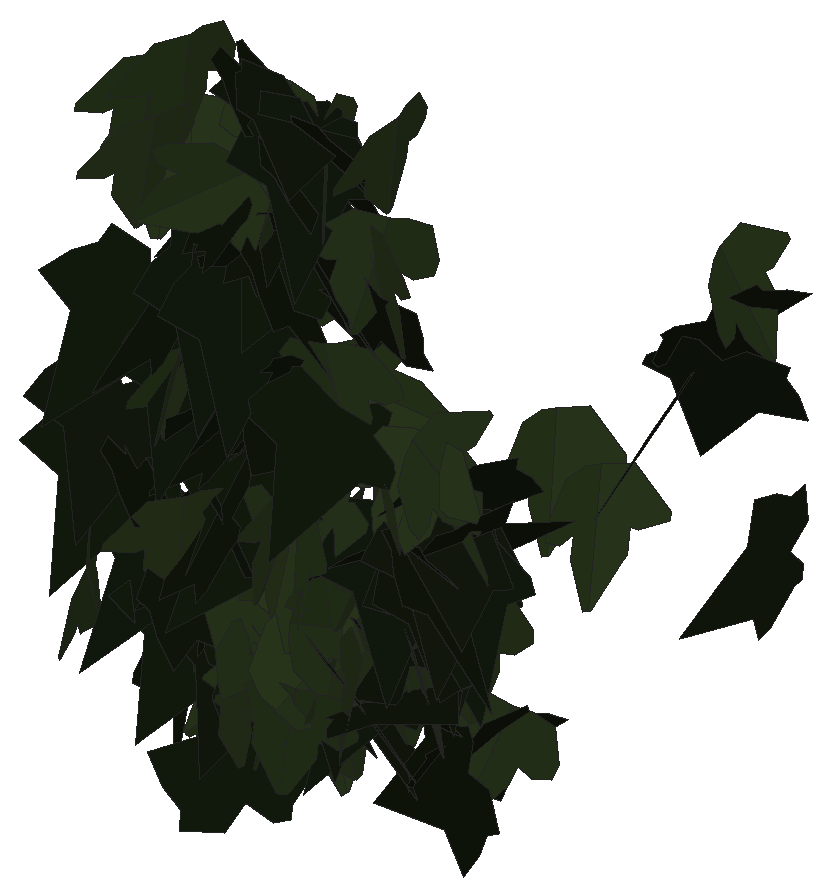
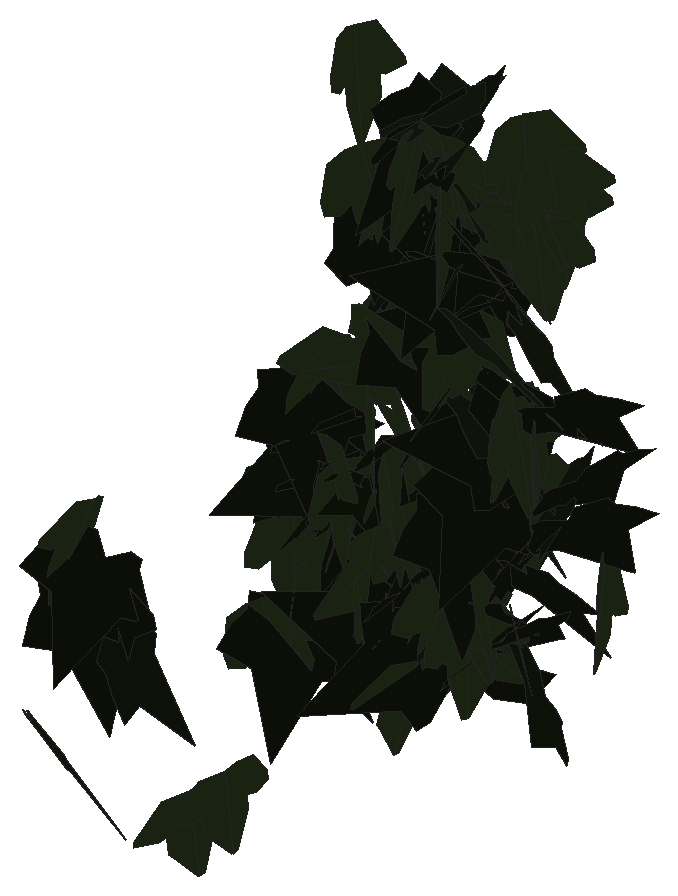
# SketchUp Ruby script. Lengths in inches.
U = 1.inch
M = Sketchup.active_model
def pt(a) = Geom::Point3d.new(a.map { |v| v * U })
def face(e, loops, mat)
  f = e.add_face(loops[0].map { |a| pt(a) })
  loops[1..].each { |l| e.add_face(l.map { |a| pt(a) }).erase! }
  f.material = f.back_material = mat if mat
  f
end
# faces: each face lists its corners as indices into pts; further lists are holes
def faces(e, pts, list, mat = nil) = list.each { |f| face(e, (f[0].is_a?(Array) ? f : [f]).map { |l| l.map { |i| pts[i] } }, mat) }
# xy, xz, yz: faces in a plane at the given z, y or x. An outline is a flat list of corners, or four numbers for a rectangle; further outlines are holes
def ring(l) = l.size == 4 ? [[l[0], l[1]], [l[2], l[1]], [l[2], l[3]], [l[0], l[3]]] : l.each_slice(2).to_a
def flat(e, list, mat, &to3) = list.each { |f| face(e, (f[0].is_a?(Array) ? f : [f]).map { |l| ring(l).map { |u, v| to3.(u, v) } }, mat) }
def xy(e, z, list, mat = nil) = flat(e, list, mat) { |x, y| [x, y, z] }
def xz(e, y, list, mat = nil) = flat(e, list, mat) { |x, z| [x, y, z] }
def yz(e, x, list, mat = nil) = flat(e, list, mat) { |y, z| [x, y, z] }
def lines(e, pts, list) = list.each { |a, b| e.add_line(pt(pts[a]), pt(pts[b])) }
# prism: a flat outline (further loops are holes) pulled along v
def prism(e, loops, v, mat = nil)
  f = face(e, loops, mat); d = Geom::Vector3d.new(v.map { |x| x * U })
  f.pushpull(f.normal.samedirection?(d) ? d.length : -d.length)
end
def box(e, o, s, mat = nil) = prism(e, [[o, [o[0] + s[0], o[1], o[2]], [o[0] + s[0], o[1] + s[1], o[2]], [o[0], o[1] + s[1], o[2]]]], [0, 0, s[2]], mat)
def at(x, y, z, deg = 0) = Geom::Transformation.translation(pt([x, y, z])) * Geom::Transformation.rotation(ORIGIN, Z_AXIS, deg.degrees)
def axes(o, x, y, z) = Geom::Transformation.new([*x, 0, *y, 0, *z, 0, *pt(o).to_a, 1])
def part(name) = M.definitions.add(name)
# library, detail: a bought-in or finely detailed component or shape, given as its bounding box
def library(name, o, s) = part(name).tap { |d| box(d.entities, o, s) }
def detail(e, o, s) = box(e.add_group.entities, o, s)
def put(e, d, t, mat = nil) = e.add_instance(d, t).tap { |i| i.material = mat if mat }
def group(e, t, mat = nil) = e.add_group.tap { |g| g.transformation = t; g.material = mat if mat }.entities
root = M.entities
M.materials.add("efeu1").color = [18, 25, 13]
M.materials.add("efeu2").color = [43, 57, 29]
c1 = part("ivyleaf_9")
p = [[1.54,2.16,1.25],[1.36,2.04,1.19],[-0.21,0.99,0.68],[-0.71,1.11,0.82],[-0.85,0.86,0.67],[-0.8,0.17,0.21],
  [-0.9,-0.01,0.1],[-0.67,-0.16,-0.02],[-0.08,-0.08,-0.05],[-0.03,-0.6,-0.4],[0.65,-0.88,-0.66],[0.83,-0.6,-0.49],
  [1.29,-0.42,-0.43],[1.8125,-0.07,-0.26],[1.21,0.44,0.15]]
faces(c1.entities,p,[[0,1,2,3,4,5,6,7,8,9,10,11,12,13,14]],"efeu1")
c2 = part("ivyleaf_10")
p = [[0,0.5,-0.03],[-0.0625,2.02,-0.43],[-0.19,2.01,-0.46],[-0.54,1.05,-0.29],[-0.52,0.625,-0.18],[-0.83,0.76,-0.28],
  [-1.16,0.64,-0.33],[-1.15,0.33,-0.24],[-0.77,-0.39,0.02],[-0.3,-0.51,0.16],[0.04,-0.48,0.23],[-0.02,2.01,-0.4375],
  [-0.06,2.01,-0.43],[0.04,-0.49,0.23],[0.67,-0.49,0.14],[1.38,0.36,-0.2],[1.375,0.51,-0.24],[0.81,0.65,-0.19],
  [0.62,0.59,-0.15],[0.6,1.09,-0.28],[0.5,1.23,-0.31]]
faces(c2.entities,p,[[0,1,2,3,4,5,6,7,8,9,10],[11,12,0,13,14,15,16,17,18,19,20]],"efeu2")
put(root,c1,axes([45.125,222.38,245.66],[-0.38766,-0.3113,0.05304],[-0.02008,-0.05951,-0.49604],[0.31515,-0.38672,0.03364]))
put(root,c1,axes([45.24,222.48,242.16],[0.00287,0.24206,0.43749],[-0.08751,0.43099,-0.23788],[-0.49227,-0.0752,0.04484]))
put(root,c1,axes([45.08,222.2,244.22],[-0.31267,-0.3897,0.01922],[-0.01187,-0.01511,-0.49963],[0.38999,-0.3129,0.0002]))
put(root,c2,axes([45.15,221.53,243.23],[0.12994,-0.37779,-0.30066],[-0.03557,0.30302,-0.39613],[0.48151,0.12433,0.05187]))
put(root,c1,axes([45.03,222.16,244.73],[-0.14946,-0.4697,0.08394],[0.01749,-0.0933,-0.49091],[0.47682,-0.14381,0.04432]))
put(root,c1,axes([45.55,222.3125,243.43],[-0.48425,-0.08758,-0.08849],[0.09295,-0.01792,-0.49096],[0.08282,-0.49194,0.03364]))
put(root,c2,axes([45.54,221.95,248.12],[-0.1573,-0.47311,0.03769],[0.00614,-0.04173,-0.49822],[0.47457,-0.15628,0.01894]))
put(root,c1,axes([45.38,221.88,244.28],[0.37177,-0.32094,-0.09373],[-0.06614,0.0668,-0.49108],[0.32774,0.37754,0.00721]))
put(root,c2,axes([45.7,222.07,245.29],[0.21508,-0.38398,-0.23728],[-0.05459,0.23878,-0.43589],[0.44806,0.21341,0.06079]))
put(root,c2,axes([45.62,222.12,247.48],[0.44327,0.22883,-0.03391],[-0.0732,0.06922,-0.48975],[-0.21944,0.43914,0.09487]))
put(root,c2,axes([45.74,222.29,245.22],[-0.05903,-0.49638,0.01103],[0.00533,-0.01174,-0.49983],[0.49648,-0.05889,0.00667]))
put(root,c2,axes([45.75,221.68,247.7],[-0.13253,-0.4821,0.00445],[-0.00203,-0.00406,-0.49998],[0.48211,-0.13254,-0.00088]))
put(root,c1,axes([45.5625,222.47,242.6],[-0.22696,0.01463,-0.44528],[0.4344,-0.10371,-0.22482],[-0.09894,-0.48891,0.03437]))
put(root,c1,axes([45.94,221.9,246.1],[-0.41221,0.27163,-0.07936],[0.06022,-0.05282,-0.49354],[-0.27651,-0.41645,0.01083]))
put(root,c1,axes([45.76,222.47,242.68],[-0.23718,-0.41431,0.14863],[0.02717,-0.18229,-0.46479],[0.43933,-0.2124,0.10898]))
put(root,c2,axes([45.93,221.93,248.46],[-0.16446,-0.47135,-0.02792],[0.01134,0.02562,-0.49921],[0.47204,-0.16483,0.00227]))
put(root,c2,axes([45.79,222.16,247.61],[0.45358,0.20748,0.03487],[0.03418,0.0091,-0.49875],[-0.20759,0.45483,-0.00592]))
put(root,c1,axes([45.875,222.17,245.54],[-0.39092,-0.19237,-0.24531],[0.24802,0.04645,-0.43166],[0.18886,-0.45917,0.05911]))
put(root,c2,axes([45.9,222.18,245.3125],[0.07023,-0.46333,-0.17432],[0.09002,0.18509,-0.45567],[0.48679,0.03262,0.10942]))
put(root,c2,axes([46.25,222.57,243.09],[-0.28832,0.05676,0.40453],[-0.39048,0.10714,-0.29334],[-0.11998,-0.48508,-0.01746]))
put(root,c1,axes([46.34,222.36,246.19],[-0.38197,0.30566,0.1033],[-0.12891,0.00218,-0.48309],[-0.29577,-0.39569,0.07714]))
put(root,c1,axes([45.9,221.86,243.44],[0.25463,-0.22596,-0.3662],[-0.18364,0.32775,-0.32993],[0.38915,0.30252,0.08392]))
put(root,c2,axes([46.11,221.66,244.11],[-0.24677,-0.43476,-0.00936],[0.00286,0.00914,-0.49991],[0.43485,-0.24678,-0.00203]))
put(root,c2,axes([46.12,222.66,242.8125],[-0.20305,-0.45486,-0.0433],[0.02949,0.03424,-0.49795],[0.45596,-0.20477,0.01293]))
put(root,c1,axes([46.14,222.26,244.25],[0.17083,0.45348,0.12318],[0.04347,0.11525,-0.48459],[-0.4679,0.17627,-0.00005]))
put(root,c1,axes([46.05,222.61,242.41],[-0.08781,-0.44591,0.20846],[0.00845,-0.21308,-0.45224],[0.49216,-0.0759,0.04495]))
put(root,c2,axes([46.16,226.73,242.65],[0.15622,0.46568,-0.09349],[-0.04238,-0.08436,-0.49101],[-0.47308,0.16133,0.01311]))
put(root,c1,axes([46.51,222.05,245.05],[-0.37045,0.32819,-0.07112],[0.0024,-0.1033,-0.48921],[-0.3358,-0.3628,0.07496]))
put(root,c2,axes([46.57,221.68,247.53],[0.27567,0.13123,-0.39596],[-0.41325,0.02121,-0.28067],[-0.05687,0.482,0.12016]))
put(root,c1,axes([46.03,222.02,244.69],[0.24987,0.03001,0.43205],[0.35568,0.27036,-0.22449],[-0.24709,0.41953,0.11376]))
put(root,c2,axes([46.5,222.46,242.52],[-0.1614,-0.27023,0.38849],[-0.1581,-0.35609,-0.31337],[0.44604,-0.224,0.0295]))
put(root,c1,axes([46.58,221.7,244.21],[-0.41189,0.28046,-0.04105],[0.03643,-0.01943,-0.49829],[-0.2811,-0.41348,-0.00443]))
put(root,c1,axes([46.625,221.86,247.375],[-0.37652,0.32747,0.03162],[-0.02185,0.02306,-0.49899],[-0.32826,-0.37714,-0.00305]))
put(root,c1,axes([46.47,222.29,243.75],[0.08376,0.48732,-0.0742],[-0.01901,-0.07201,-0.49442],[-0.49257,0.08565,0.00647]))
put(root,c2,axes([46.4,222.65,242.98],[-0.34952,-0.35193,-0.06307],[0.0779,0.01113,-0.49377],[0.34895,-0.35499,0.04705]))
put(root,c2,axes([46.36,222.15,242.64],[-0.3735,0.31157,-0.11585],[0.07852,-0.08663,-0.48614],[-0.323,-0.38134,0.01579]))
put(root,c1,axes([46.375,222.57,242.81],[-0.32423,-0.35122,-0.14671],[0.12402,0.08472,-0.47691],[0.35985,-0.34564,0.03218]))
put(root,c1,axes([46.3125,222.01,246.38],[-0.10842,-0.48688,0.03449],[0.01245,-0.03808,-0.49839],[0.48795,-0.10721,0.02038]))
put(root,c1,axes([46.79,222.1,247.15],[-0.47088,0.16808,0.00458],[-0.00322,0.00463,-0.49997],[-0.16811,-0.47088,-0.00328]))
put(root,c2,axes([46.49,222.27,246.1],[-0.44192,-0.17527,-0.15488],[0.15416,0.03071,-0.47465],[0.17589,-0.46727,0.0269]))
put(root,c1,axes([46.32,222.22,243.91],[0.37188,-0.33039,-0.05049],[-0.03501,0.03661,-0.49743],[0.33238,0.3735,0.0041]))
put(root,c1,axes([46.71,221.77,241.53],[-0.46663,-0.08066,0.16047],[0.15811,0.0274,0.47355],[-0.08518,0.49269,-0.00007]))
put(root,c1,axes([46.81,222.09,244.27],[-0.46675,-0.1788,0.01334],[-0.01132,-0.00773,-0.49981],[0.17894,-0.46687,0.00316]))
put(root,c2,axes([46.62,226.76,242.25],[0.17252,0.46016,-0.09213],[-0.05885,-0.07617,-0.49065],[-0.46559,0.18014,0.02788]))
put(root,c1,axes([46.78,222.23,246.78],[-0.44314,-0.22095,-0.06932],[0.0776,-0.00068,-0.49394],[0.21818,-0.44853,0.03489]))
put(root,c2,axes([46.74,222.49,242.58],[-0.00841,0.42234,-0.2675],[-0.11132,-0.2624,-0.4108],[-0.48738,0.05265,0.09845]))
put(root,c1,axes([46.61,221.9375,246.36],[-0.08779,-0.49219,0.00671],[0.00137,-0.00706,-0.49995],[0.49223,-0.08777,0.00259]))
put(root,c1,axes([46.43,222.0625,246.41],[0.23802,-0.01532,0.43944],[0.38697,0.2446,-0.20107],[-0.20881,0.43582,0.12829]))
put(root,c1,axes([46.54,222.49,242.83],[0.38172,-0.27841,-0.16365],[-0.09931,0.1399,-0.46964],[0.30729,0.39105,0.0515]))
put(root,c2,axes([46.68,222.94,242.11],[0.12285,0.4826,0.04481],[0.00308,0.04545,-0.49792],[-0.48466,0.12262,0.00819]))
put(root,c2,axes([46.77,222.27,247.44],[0.1814,-0.44126,-0.14962],[0.03193,0.17196,-0.46841],[0.46484,0.16039,0.09057]))
put(root,c1,axes([46.72,221.94,246.99],[0.40306,0.29273,-0.04303],[-0.04329,-0.01359,-0.49794],[-0.29269,0.40512,0.01439]))
put(root,c2,axes([46.81,221.47,242.71],[0.11259,-0.12417,-0.47107],[0.05349,0.48371,-0.11472],[0.48421,-0.02456,0.1222]))
put(root,c2,axes([46.95,221.8,244.16],[0.35532,-0.25677,-0.24046],[-0.18313,0.1568,-0.43804],[0.30036,0.39935,0.01738]))
put(root,c1,axes([46.55,222.88,242.36],[0.37762,0.19109,0.26625],[0.24386,0.10753,-0.42305],[-0.21894,0.44936,-0.01199]))
put(root,c1,axes([46.59,221.92,248.5],[0.36501,-0.33331,-0.0753],[-0.04206,0.06552,-0.4939],[0.33911,0.36689,0.01979]))
put(root,c2,axes([46.8,222.15,248.11],[0.49516,-0.06937,-0.00223],[-0.00279,-0.00384,-0.49998],[0.06935,0.49515,-0.00419]))
put(root,c2,axes([46.59,221.97,243.38],[-0.24818,-0.17193,-0.39856],[0.42152,0.01409,-0.26855],[0.10358,-0.4693,0.13795]))
put(root,c1,axes([46.73,222.1875,245.24],[0.2571,-0.3921,-0.17365],[-0.09116,0.14787,-0.46886],[0.41903,0.27275,0.00454]))
put(root,c2,axes([46.99,222.6,243.63],[-0.17064,-0.46105,0.09119],[0.00281,-0.09801,-0.49029],[0.46997,-0.16681,0.03604]))
put(root,c1,axes([46.8,222,246.73],[0.36307,-0.31106,-0.14636],[-0.11129,0.09506,-0.4781],[0.32526,0.37974,-0.0002]))
put(root,c1,axes([47.19,222.11,245.75],[0.07986,0.44036,-0.22294],[-0.08151,-0.21097,-0.44592],[-0.4868,0.10757,0.03809]))
put(root,c2,axes([47.22,221.82,242.55],[-0.43911,-0.21466,0.10538],[-0.09298,-0.04972,-0.48876],[0.22031,-0.44883,0.00375]))
put(root,c2,axes([47.125,222.5,242.27],[-0.16151,-0.44852,-0.15081],[0.05772,0.13948,-0.47667],[0.46966,-0.17138,0.00672]))
put(root,c1,axes([46.96,222.73,242.94],[-0.00201,-0.49969,0.01762],[0.00168,-0.01763,-0.49969],[0.49999,-0.00195,0.00175]))
put(root,c2,axes([47.19,221.84,244.55],[0.07256,-0.47846,0.12574],[0.00556,-0.12629,-0.48376],[0.49468,0.0716,-0.013]))
put(root,c2,axes([47.22,222.2,247.92],[0.02177,-0.42929,-0.25541],[0.04832,0.25627,-0.42661],[0.49718,-0.00611,0.05265]))
put(root,c2,axes([47.25,222.55,244.16],[0.14391,-0.47643,-0.04806],[0.00429,0.05146,-0.49733],[0.47882,0.14272,0.0189]))
put(root,c2,axes([47.29,222.41,242.8],[0.15196,-0.4738,-0.04919],[0.01479,0.0563,-0.4966],[0.47612,0.14947,0.03112]))
put(root,c2,axes([47.32,222.89,242.86],[0.13243,-0.47499,-0.08272],[0.00013,0.08582,-0.49258],[0.48214,0.13044,0.02285]))
put(root,c1,axes([47.04,222.91,242.53],[0.23949,-0.43726,-0.03809],[0.01293,0.0504,-0.49729],[0.43872,0.2372,0.03545]))
put(root,c1,axes([47.09,222.04,248.3125],[-0.12571,-0.43276,0.21661],[0.23524,-0.25022,-0.36339],[0.42292,0.01055,0.26651]))
put(root,c2,axes([47.15,221.86,244.21],[0.44446,-0.15156,0.17172],[0.1627,-0.05492,-0.46959],[0.1612,0.4733,0.00049]))
put(root,c2,axes([47.22,222.72,243.29],[-0.04241,-0.21685,-0.44853],[0.20092,0.40448,-0.21455],[0.45589,-0.19843,0.05283]))
put(root,c1,axes([47.17,221.7,248.07],[0.40828,-0.18027,-0.22542],[-0.15091,0.19954,-0.43291],[0.24604,0.42153,0.10852]))
put(root,c1,axes([46.98,222.92,242.41],[0.13818,-0.00884,0.48045],[0.48053,0.00261,-0.13815],[-0.00007,0.49992,0.00922]))
put(root,c2,axes([47.29,222.15,244.29],[0.43164,-0.2521,0.01133],[0.00079,0.0238,0.49943],[-0.25235,-0.43114,0.02095]))
put(root,c1,axes([47.4375,222.67,243.13],[0.36662,0.14186,-0.30897],[-0.30233,-0.07182,-0.39171],[-0.15552,0.47404,0.03311]))
put(root,c1,axes([47.23,221.88,248.14],[0.4894,0.04217,-0.09332],[-0.09344,-0.00255,-0.49119],[-0.0419,0.49821,0.00538]))
put(root,c2,axes([47.43,222.07,245.87],[-0.4808,-0.12821,-0.04892],[0.05558,-0.01897,-0.49654],[0.12547,-0.48291,0.03249]))
put(root,c2,axes([47.22,221.81,242.77],[0.21004,0.22899,-0.39173],[0.26804,0.28568,0.31071],[0.36611,-0.34052,-0.00275]))
put(root,c2,axes([47.47,222.29,243.64],[-0.02929,-0.45273,0.21018],[0.02436,-0.21158,-0.45237],[0.49855,-0.01626,0.03445]))
put(root,c2,axes([47.47,221.74,243.46],[-0.03978,0.21473,0.44979],[-0.12704,0.43194,-0.21745],[-0.48195,-0.13159,0.02019]))
put(root,c2,axes([47.4,221.89,247.82],[0.38152,-0.32094,-0.038],[0.02963,0.09327,-0.49033],[0.32182,0.37189,0.09019]))
put(root,c1,axes([47.32,221.91,247.01],[0.43518,-0.15218,-0.19355],[-0.18332,0.06212,-0.46102],[0.16436,0.47221,-0.00173]))
put(root,c1,axes([47.37,221.9,248.15],[-0.08028,-0.49346,0.00712],[-0.00437,-0.00651,-0.49994],[0.49349,-0.08033,-0.00327]))
put(root,c2,axes([47.59,222.54,242.68],[-0.07579,-0.45832,0.18493],[-0.04263,-0.18033,-0.46439],[0.49238,-0.08616,-0.01175]))
put(root,c1,axes([47.51,222.1,245.41],[-0.23957,-0.43175,0.07874],[-0.03548,-0.07036,-0.49375],[0.43743,-0.24217,0.00308]))
put(root,c1,axes([47.12,222.71,242.64],[0.28177,-0.19771,0.36265],[0.29187,-0.21532,-0.34416],[0.29226,0.40564,-0.00593]))
put(root,c1,axes([47.65,226.61,243.74],[-0.3171,0.26075,-0.28541],[0.17579,-0.23151,-0.40682],[-0.34431,-0.35835,0.05515]))
put(root,c1,axes([47.77,222.29,244.05],[-0.04574,0.47551,-0.14765],[-0.11941,-0.15443,-0.46032],[-0.48337,-0.00685,0.12769]))
put(root,c1,axes([47.65,222.63,242.89],[-0.47782,-0.07937,-0.12406],[0.12722,-0.0102,-0.48344],[0.07421,-0.49355,0.02995]))
put(root,c1,axes([47.22,222.2,242.92],[0.34801,-0.3038,0.1913],[0.13837,-0.13233,-0.46189],[0.33127,0.37442,-0.00803]))
put(root,c2,axes([47.78,222.3,244.67],[-0.35823,0.31771,0.14397],[-0.17966,0.00883,-0.46652],[-0.29898,-0.38598,0.10784]))
put(root,c2,axes([47.76,222.64,243.94],[-0.1562,-0.47349,-0.03753],[0.0053,0.03776,-0.49854],[0.47495,-0.15614,-0.00678]))
put(root,c2,axes([47.375,222.41,245.48],[0.10079,0.07589,0.48382],[0.39596,0.27806,-0.1261],[-0.2882,0.40856,-0.00404]))
put(root,c1,axes([48.07,222.31,243.09],[-0.06093,0.25404,0.42632],[-0.28103,0.33635,-0.2406],[-0.40903,-0.26894,0.1018]))
put(root,c1,axes([47.86,222.16,246.27],[0.3084,-0.2148,0.32978],[-0.2742,0.18327,0.3758],[-0.28232,-0.41264,-0.00476]))
put(root,c1,axes([47.73,222.33,244.04],[0.43139,0.17913,-0.17837],[-0.17166,-0.05141,-0.46679],[-0.18557,0.46397,0.01715]))
put(root,c2,axes([47.875,222.38,243.08],[-0.49771,-0.04269,0.02144],[-0.02117,-0.00414,-0.49953],[0.04283,-0.49816,0.00232]))
put(root,c1,axes([47.76,222.53,244.07],[-0.05078,-0.4971,-0.01767],[-0.0052,0.01829,-0.49964],[0.49739,-0.05056,-0.00703]))
put(root,c2,axes([47.95,221.69,243.16],[0.28344,-0.36878,-0.18347],[-0.06707,0.17842,-0.46224],[0.4064,0.28665,0.05167]))
put(root,c2,axes([47.95,222.7,243.07],[-0.01111,0.32085,0.38332],[-0.1247,0.36951,-0.31291],[-0.48407,-0.10256,0.07181]))
put(root,c2,axes([48.0625,221.97,247.38],[-0.32864,-0.35008,0.13943],[-0.06618,-0.12851,-0.47865],[0.37097,-0.33306,0.03813]))
put(root,c1,axes([48.11,226.56,244.14],[0.24966,0.29695,-0.31542],[-0.2338,-0.21412,-0.38664],[-0.3647,0.34055,0.03194]))
put(root,c2,axes([48.07,222.73,244.18],[-0.48402,0.1152,0.04957],[-0.06808,-0.0754,-0.48957],[-0.10533,-0.48067,0.08868]))
put(root,c2,axes([47.96,221.97,247.27],[-0.39053,0.29127,-0.11245],[0.08013,-0.08055,-0.48692],[-0.30177,-0.39834,0.01623]))
put(root,c1,axes([48.04,226.48,244.57],[0.21491,0.4485,0.05156],[0.01669,0.04918,-0.4973],[-0.45115,0.21547,0.00617]))
put(root,c2,axes([48.15,222.35,245.04],[0.48147,0.09797,-0.09269],[-0.08788,-0.03276,-0.49113],[-0.10231,0.48921,-0.01432]))
put(root,c2,axes([48.16,222.31,243.22],[-0.2994,0.40025,0.01261],[-0.00591,0.01133,-0.49984],[-0.40041,-0.29945,-0.00205]))
put(root,c1,axes([47.98,222.78,243.71],[0.10296,-0.48698,0.04737],[0.01021,-0.04626,-0.49775],[0.48918,0.10347,0.00042]))
put(root,c1,axes([48.54,222.5,242.05],[0.0111,-0.0115,-0.49974],[-0.47754,-0.14799,-0.0072],[-0.14775,0.47746,-0.01427]))
put(root,c1,axes([48.3,222.9,242.09],[0.14383,0.47872,-0.01179],[-0.01201,-0.00869,-0.49978],[-0.47871,0.14405,0.009]))
put(root,c1,axes([48.35,222.56,244.77],[0.1301,0.4554,-0.16026],[-0.05087,-0.15212,-0.47357],[-0.48009,0.13953,0.00675]))
put(root,c1,axes([48.15,222.79,243.89],[-0.07605,-0.48117,-0.11267],[-0.00092,0.11413,-0.4868],[0.49418,-0.07384,-0.01824]))
put(root,c2,axes([48.23,226.58,245.09],[-0.07238,0.46697,0.16342],[-0.02156,0.16202,-0.47253],[-0.49426,-0.07545,-0.00332]))
put(root,c2,axes([48.36,221.73,248.61],[-0.01721,-0.48825,-0.10639],[-0.01373,0.10687,-0.48825],[0.49952,-0.01388,-0.01709]))
put(root,c2,axes([48.47,223.13,242.23],[-0.4034,-0.21842,0.19891],[-0.12927,-0.17221,-0.45126],[0.26563,-0.4155,0.08247]))
put(root,c1,axes([48.18,222.59,243.99],[0.27314,0.22404,0.35384],[0.19426,0.30647,-0.34401],[-0.37102,0.3254,0.08037]))
put(root,c2,axes([48.38,222.8,243.28],[-0.27945,-0.41446,-0.0112],[0.02168,-0.00112,-0.49953],[0.41405,-0.27967,0.0186]))
put(root,c1,axes([48.22,222.75,243.95],[-0.25774,-0.27188,-0.33114],[0.21531,0.25191,-0.37441],[0.37042,-0.3356,-0.01278]))
put(root,c2,axes([48.34,222.27,245.16],[0.01443,0.41306,0.28138],[-0.04265,0.28149,-0.41103],[-0.49797,-0.01214,0.04336]))
put(root,c1,axes([48.125,222.43,244.0625],[0.29935,-0.40049,0.00149],[0.00091,-0.00118,-0.5],[0.40049,0.29935,0.00002]))
put(root,c1,axes([48.05,222.18,242.75],[0.01292,-0.4943,0.07416],[0.48859,-0.00315,-0.10615],[0.10541,0.07521,0.48294]))
put(root,c1,axes([48.3,222.66,244.29],[-0.12005,-0.48327,-0.04511],[0.01369,0.04308,-0.49795],[0.48518,-0.12079,0.00289]))
put(root,c1,axes([48.68,226.71,242.41],[-0.44725,0.22346,0.00529],[-0.0055,0.00083,-0.49997],[-0.22346,-0.44729,0.00171]))
